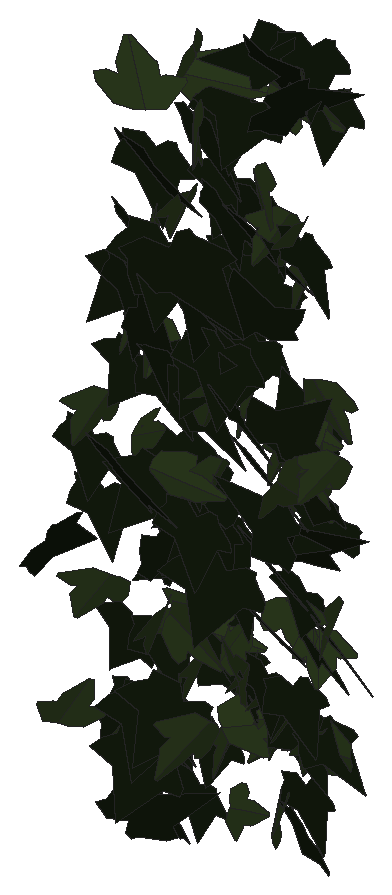
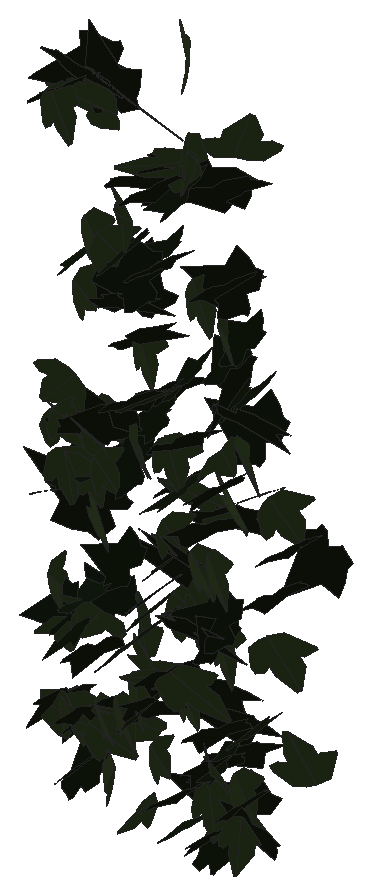
# SketchUp Ruby script. Lengths in inches.
U = 1.inch
M = Sketchup.active_model
def pt(a) = Geom::Point3d.new(a.map { |v| v * U })
def face(e, loops, mat)
  f = e.add_face(loops[0].map { |a| pt(a) })
  loops[1..].each { |l| e.add_face(l.map { |a| pt(a) }).erase! }
  f.material = f.back_material = mat if mat
  f
end
# faces: each face lists its corners as indices into pts; further lists are holes
def faces(e, pts, list, mat = nil) = list.each { |f| face(e, (f[0].is_a?(Array) ? f : [f]).map { |l| l.map { |i| pts[i] } }, mat) }
# xy, xz, yz: faces in a plane at the given z, y or x. An outline is a flat list of corners, or four numbers for a rectangle; further outlines are holes
def ring(l) = l.size == 4 ? [[l[0], l[1]], [l[2], l[1]], [l[2], l[3]], [l[0], l[3]]] : l.each_slice(2).to_a
def flat(e, list, mat, &to3) = list.each { |f| face(e, (f[0].is_a?(Array) ? f : [f]).map { |l| ring(l).map { |u, v| to3.(u, v) } }, mat) }
def xy(e, z, list, mat = nil) = flat(e, list, mat) { |x, y| [x, y, z] }
def xz(e, y, list, mat = nil) = flat(e, list, mat) { |x, z| [x, y, z] }
def yz(e, x, list, mat = nil) = flat(e, list, mat) { |y, z| [x, y, z] }
def lines(e, pts, list) = list.each { |a, b| e.add_line(pt(pts[a]), pt(pts[b])) }
# prism: a flat outline (further loops are holes) pulled along v
def prism(e, loops, v, mat = nil)
  f = face(e, loops, mat); d = Geom::Vector3d.new(v.map { |x| x * U })
  f.pushpull(f.normal.samedirection?(d) ? d.length : -d.length)
end
def box(e, o, s, mat = nil) = prism(e, [[o, [o[0] + s[0], o[1], o[2]], [o[0] + s[0], o[1] + s[1], o[2]], [o[0], o[1] + s[1], o[2]]]], [0, 0, s[2]], mat)
def at(x, y, z, deg = 0) = Geom::Transformation.translation(pt([x, y, z])) * Geom::Transformation.rotation(ORIGIN, Z_AXIS, deg.degrees)
def axes(o, x, y, z) = Geom::Transformation.new([*x, 0, *y, 0, *z, 0, *pt(o).to_a, 1])
def part(name) = M.definitions.add(name)
# library, detail: a bought-in or finely detailed component or shape, given as its bounding box
def library(name, o, s) = part(name).tap { |d| box(d.entities, o, s) }
def detail(e, o, s) = box(e.add_group.entities, o, s)
def put(e, d, t, mat = nil) = e.add_instance(d, t).tap { |i| i.material = mat if mat }
def group(e, t, mat = nil) = e.add_group.tap { |g| g.transformation = t; g.material = mat if mat }.entities
root = M.entities
M.materials.add("1026 AP 7946 SUNNY SIDE UP").color = [254, 231, 186]
M.materials.add("efeu1").color = [18, 25, 13]
M.materials.add("efeu2").color = [43, 57, 29]
c1 = part("ivyleaf_10")
p = [[0,0.5,-0.03],[-0.0625,2.02,-0.43],[-0.19,2.01,-0.46],[-0.54,1.05,-0.29],[-0.52,0.625,-0.18],[-0.83,0.76,-0.28],
  [-1.16,0.64,-0.33],[-1.15,0.33,-0.24],[-0.77,-0.39,0.02],[-0.3,-0.51,0.16],[0.04,-0.48,0.23],[-0.02,2.01,-0.4375],
  [-0.06,2.01,-0.43],[0.04,-0.49,0.23],[0.67,-0.49,0.14],[1.38,0.36,-0.2],[1.375,0.51,-0.24],[0.81,0.65,-0.19],
  [0.62,0.59,-0.15],[0.6,1.09,-0.28],[0.5,1.23,-0.31]]
faces(c1.entities,p,[[0,1,2,3,4,5,6,7,8,9,10],[11,12,0,13,14,15,16,17,18,19,20]],"efeu2")
c2 = part("ivyleaf_9")
p = [[1.54,2.16,1.25],[1.36,2.04,1.19],[-0.21,0.99,0.68],[-0.71,1.11,0.82],[-0.85,0.86,0.67],[-0.8,0.17,0.21],
  [-0.9,-0.01,0.1],[-0.67,-0.16,-0.02],[-0.08,-0.08,-0.05],[-0.03,-0.6,-0.4],[0.65,-0.88,-0.66],[0.83,-0.6,-0.49],
  [1.29,-0.42,-0.43],[1.8125,-0.07,-0.26],[1.21,0.44,0.15]]
faces(c2.entities,p,[[0,1,2,3,4,5,6,7,8,9,10,11,12,13,14]],"efeu1")
put(root,c1,axes([104.9,211.85,273.21],[-0.13637,-0.25929,0.15931],[-0.00882,-0.16099,-0.27962],[0.47582,-0.0773,0.04048]),"1026 AP 7946 SUNNY SIDE UP")
put(root,c2,axes([104.76,211.88,272.62],[-0.08872,-0.27066,0.06287],[-0.00066,-0.06376,-0.28492],[0.43681,-0.05507,0.01234]),"1026 AP 7946 SUNNY SIDE UP")
put(root,c1,axes([104.85,211.24,268.93],[-0.23309,-0.23778,0.08634],[0.05181,0.07969,0.28879],[-0.39375,0.15124,-0.01311]),"1026 AP 7946 SUNNY SIDE UP")
put(root,c2,axes([105.06,212.45,274.85],[-0.44652,-0.06542,-0.02912],[0.05355,-0.02432,-0.29862],[0.09817,-0.2843,0.03048]),"1026 AP 7946 SUNNY SIDE UP")
put(root,c1,axes([105.03,212.42,274.24],[0.21825,-0.25056,0.01931],[-0.00739,-0.02562,-0.29475],[0.39519,0.1379,-0.01618]),"1026 AP 7946 SUNNY SIDE UP")
put(root,c2,axes([104.9375,211.88,271.9],[-0.04719,-0.27806,-0.01852],[0.00454,0.01618,-0.28802],[0.43795,-0.03013,0.00099]),"1026 AP 7946 SUNNY SIDE UP")
put(root,c2,axes([105.04,212.46,273.54],[-0.21801,-0.20803,0.13532],[-0.01162,-0.14847,-0.2489],[0.38767,-0.12144,0.06864]),"1026 AP 7946 SUNNY SIDE UP")
put(root,c1,axes([105.2,211.54,270.84],[-0.2765,-0.20385,0.12948],[-0.11042,-0.10669,-0.27754],[0.36102,-0.18876,0.01429]),"1026 AP 7946 SUNNY SIDE UP")
put(root,c1,axes([105.15,212.29,268.43],[-0.15989,-0.26875,-0.07973],[0.05518,0.0678,-0.2955],[0.43562,-0.10723,0.00817]),"1026 AP 7946 SUNNY SIDE UP")
put(root,c2,axes([105.17,210.46,271.89],[-0.08244,0.06946,-0.3413],[-0.20675,0.30517,0.08904],[0.49112,0.14013,-0.01981]),"1026 AP 7946 SUNNY SIDE UP")
put(root,c2,axes([105.11,212.25,269.82],[-0.12855,-0.20054,0.19397],[-0.03349,-0.19239,-0.22043],[0.43247,-0.07451,0.04059]),"1026 AP 7946 SUNNY SIDE UP")
put(root,c2,axes([105.09,212.36,268.85],[0.03221,-0.26751,-0.0102],[-0.01043,0.0079,-0.27627],[0.4207,0.02068,-0.00607]),"1026 AP 7946 SUNNY SIDE UP")
put(root,c2,axes([105.14,212.16,274.92],[0.02183,-0.27141,0.12572],[0.00089,-0.12368,-0.28064],[0.46892,0.01287,-0.00532]),"1026 AP 7946 SUNNY SIDE UP")
put(root,c2,axes([105.0625,212.2,268.5],[-0.13577,-0.09502,-0.25981],[0.39493,0.06615,-0.11412],[0.15144,-0.2577,0.06469]),"1026 AP 7946 SUNNY SIDE UP")
put(root,c1,axes([105.38,212.03,268.92],[0.00367,-0.26318,0.05046],[0.00058,-0.05047,-0.27143],[0.42137,0.00236,-0.00007]),"1026 AP 7946 SUNNY SIDE UP")
put(root,c1,axes([105.36,212.4375,274.15],[0.09008,0.24911,-0.15821],[-0.05799,-0.15054,-0.26421],[-0.45767,0.06811,0.00234]),"1026 AP 7946 SUNNY SIDE UP")
put(root,c2,axes([105.33,212.42,276.71],[-0.07345,-0.30952,-0.02113],[0.01188,0.01782,-0.32233],[0.48744,-0.04708,0.00468]),"1026 AP 7946 SUNNY SIDE UP")
put(root,c2,axes([105.21,212.15,275.69],[0.09186,-0.2163,0.20667],[0.10874,-0.19006,-0.23155],[0.45231,0.08962,0.0137]),"1026 AP 7946 SUNNY SIDE UP")
put(root,c2,axes([105.14,212.27,276.61],[0.27502,-0.1664,0.2202],[0.20993,-0.16971,-0.24855],[0.37195,0.21882,-0.02254]),"1026 AP 7946 SUNNY SIDE UP")
put(root,c1,axes([105.64,212.27,272.25],[0.0843,-0.28218,-0.00006],[-0.00823,-0.00256,-0.29586],[0.44363,0.05358,-0.00548]),"1026 AP 7946 SUNNY SIDE UP")
put(root,c2,axes([105.4375,212.4375,273.6],[0.05174,-0.275,-0.07016],[0.01303,0.0679,-0.28446],[0.4447,0.03001,0.0165]),"1026 AP 7946 SUNNY SIDE UP")
put(root,c2,axes([105.49,212.38,269.87],[-0.04198,-0.26855,-0.07003],[0.0351,0.06445,-0.27719],[0.43359,-0.03122,0.01566]),"1026 AP 7946 SUNNY SIDE UP")
put(root,c1,axes([105.47,212.28,275.92],[0.17667,-0.18158,0.26379],[0.25223,-0.20184,-0.22026],[0.42582,0.1949,0.02102]),"1026 AP 7946 SUNNY SIDE UP")
put(root,c2,axes([105.48,212.4,268.3125],[0.08229,-0.24938,-0.08234],[0.01437,0.08177,-0.26081],[0.41086,0.04709,0.02562]),"1026 AP 7946 SUNNY SIDE UP")
put(root,c1,axes([105.7,212.25,268.74],[-0.12518,-0.28862,-0.03169],[0.02286,0.0262,-0.3082],[0.45556,-0.08062,0.00676]),"1026 AP 7946 SUNNY SIDE UP")
put(root,c2,axes([105.44,212.18,275.33],[0.03713,-0.23221,0.2238],[0.08523,-0.21305,-0.24047],[0.49412,0.0542,0.02466]),"1026 AP 7946 SUNNY SIDE UP")
put(root,c2,axes([105.6875,212.09,270.97],[-0.11798,-0.09311,0.30162],[0.27453,0.23574,0.12448],[-0.39848,0.18998,-0.00354]),"1026 AP 7946 SUNNY SIDE UP")
put(root,c2,axes([105.35,212.36,271.51],[0.31568,-0.1769,0.16046],[0.15625,-0.12345,-0.27534],[0.33722,0.2228,-0.02264]),"1026 AP 7946 SUNNY SIDE UP")
put(root,c1,axes([105.49,211.9375,272.88],[0.09376,-0.2018,-0.22314],[0.21226,-0.17684,0.20809],[-0.41281,-0.13677,0.05632]),"1026 AP 7946 SUNNY SIDE UP")
put(root,c2,axes([105.74,211.59,274.93],[0.13813,-0.14527,-0.30319],[-0.28903,0.2296,-0.17241],[0.42613,0.20281,-0.01867]),"1026 AP 7946 SUNNY SIDE UP")
put(root,c1,axes([105.79,212.43,272.34],[0.08405,-0.26833,0.06119],[0.00277,-0.06172,-0.28203],[0.43265,0.05252,-0.01008]),"1026 AP 7946 SUNNY SIDE UP")
put(root,c1,axes([105.6,212.35,269.28],[0.27085,-0.11401,0.1883],[0.21361,-0.1252,-0.21233],[0.26401,0.21827,-0.02138]),"1026 AP 7946 SUNNY SIDE UP")
put(root,c2,axes([105.88,212.01,267.58],[0.20182,-0.28633,0.03714],[-0.00612,0.03951,0.32323],[-0.45406,-0.1278,0.01215]),"1026 AP 7946 SUNNY SIDE UP")
put(root,c1,axes([105.875,211.44,278.15],[0.38142,0.24059,0.01396],[-0.04199,0.00967,0.35102],[0.37645,-0.24268,0.02501]),"1026 AP 7946 SUNNY SIDE UP")
put(root,c1,axes([106.1875,212.32,270.33],[-0.25609,-0.06799,0.2564],[-0.33715,-0.12884,-0.18128],[0.22668,-0.26844,0.02004]),"1026 AP 7946 SUNNY SIDE UP")
put(root,c2,axes([106.11,212.41,271.28],[-0.45539,-0.01295,0.03436],[-0.05016,-0.03104,-0.2973],[0.02572,-0.28988,0.02858]),"1026 AP 7946 SUNNY SIDE UP")
put(root,c1,axes([105.9375,212.24,276.3125],[-0.00814,-0.29914,0.02278],[0.00021,-0.02382,-0.30835],[0.47185,-0.00515,0.00053]),"1026 AP 7946 SUNNY SIDE UP")
put(root,c2,axes([105.6875,211.99,269.13],[0.23262,-0.22919,-0.01236],[-0.02358,0.00304,-0.28078],[0.36,0.14829,-0.01041]),"1026 AP 7946 SUNNY SIDE UP")
put(root,c2,axes([105.71,211.8125,274.46],[0.10779,-0.26528,0.10233],[0.0118,-0.10201,-0.28231],[0.44609,0.0668,-0.01726]),"1026 AP 7946 SUNNY SIDE UP")
put(root,c2,axes([105.8,212.02,269.1],[0.00751,-0.25154,-0.10071],[0.02049,0.09645,-0.25822],[0.42304,-0.0002,0.01429]),"1026 AP 7946 SUNNY SIDE UP")
put(root,c2,axes([105.82,212.24,272.8],[-0.05672,-0.26808,-0.09466],[0.06542,0.08507,-0.27663],[0.44,-0.04721,0.02893]),"1026 AP 7946 SUNNY SIDE UP")
put(root,c2,axes([106.125,211.58,272.6],[-0.37623,-0.18071,0.05784],[-0.04976,-0.05269,-0.30833],[0.29385,-0.2403,0.02184]),"1026 AP 7946 SUNNY SIDE UP")
put(root,c1,axes([106.11,211.54,270.7],[0.04765,-0.33136,-0.03264],[-0.01071,0.0293,-0.34259],[0.52302,0.03079,-0.00404]),"1026 AP 7946 SUNNY SIDE UP")
put(root,c1,axes([106.07,212.23,278.49],[0.0481,-0.28273,-0.13279],[0.06871,0.13057,-0.28717],[0.48268,0.00959,0.05411]),"1026 AP 7946 SUNNY SIDE UP")
put(root,c2,axes([106.15,211.26,268.79],[-0.26122,-0.27364,0.06493],[-0.0318,-0.06319,-0.32979],[0.44095,-0.16667,0.01468]),"1026 AP 7946 SUNNY SIDE UP")
put(root,c2,axes([106.2,211.4,269.43],[-0.41224,-0.17388,-0.09526],[0.14983,0.02088,-0.32208],[0.27017,-0.27689,0.03327]),"1026 AP 7946 SUNNY SIDE UP")
put(root,c2,axes([106.22,212.39,274],[-0.21257,-0.24818,0.0884],[-0.0298,-0.08862,-0.29056],[0.41256,-0.13427,0.02456]),"1026 AP 7946 SUNNY SIDE UP")
put(root,c2,axes([106.02,212.4,273.36],[0.21197,-0.25152,-0.06967],[-0.00573,0.07273,-0.2919],[0.40892,0.1314,0.03202]),"1026 AP 7946 SUNNY SIDE UP")
put(root,c2,axes([106.53,212.28,272.32],[-0.49536,0.04052,-0.00725],[0.00486,-0.03261,-0.32575],[-0.06454,-0.31343,0.03107]),"1026 AP 7946 SUNNY SIDE UP")
put(root,c2,axes([105.99,211.12,267.89],[0.01157,0.00502,0.33337],[0.50166,0.05409,-0.00802],[-0.08522,0.3191,-0.00196]),"1026 AP 7946 SUNNY SIDE UP")
put(root,c2,axes([106.24,212.53,268.6],[-0.11135,-0.23911,0.07407],[-0.0032,-0.07559,-0.25662],[0.39321,-0.06833,0.01889]),"1026 AP 7946 SUNNY SIDE UP")
put(root,c2,axes([106.21,212.21,274.82],[-0.016,-0.23467,0.22372],[-0.01108,-0.21839,-0.24325],[0.50405,-0.01225,0.00175]),"1026 AP 7946 SUNNY SIDE UP")
put(root,c2,axes([106.25,212.15,267.99],[-0.05486,-0.24507,0.10833],[0.02508,-0.10917,-0.25394],[0.41943,-0.02552,0.02935]),"1026 AP 7946 SUNNY SIDE UP")
put(root,c1,axes([106.4,211.97,269.9375],[0.06799,-0.2653,0.06896],[0.02081,-0.06719,-0.2773],[0.43031,0.04517,0.00251]),"1026 AP 7946 SUNNY SIDE UP")
put(root,c1,axes([106.45,212.2,273.74],[-0.11432,-0.2791,0.02523],[0.00059,-0.02704,-0.29719],[0.44077,-0.07236,0.00694]),"1026 AP 7946 SUNNY SIDE UP")
put(root,c1,axes([106.4,212.28,272.5625],[-0.04556,-0.24319,0.14883],[0.06393,-0.14866,-0.2479],[0.44128,-0.00357,0.05128]),"1026 AP 7946 SUNNY SIDE UP")
put(root,c2,axes([106.38,212.35,270.42],[-0.0352,-0.26991,-0.06468],[0.0018,0.06136,-0.27862],[0.43519,-0.02208,-0.00408]),"1026 AP 7946 SUNNY SIDE UP")
put(root,c2,axes([106.29,212.04,277.66],[0.25695,-0.28729,0.00723],[-0.01279,-0.01457,-0.34026],[0.45176,0.16299,-0.01375]),"1026 AP 7946 SUNNY SIDE UP")
put(root,c1,axes([106.22,212.22,278.17],[-0.0047,-0.11737,-0.3196],[0.45124,0.15345,-0.0619],[0.25959,-0.26888,0.10181]),"1026 AP 7946 SUNNY SIDE UP")
put(root,c2,axes([106.49,212.55,276.63],[-0.15166,-0.26073,0.10988],[-0.02607,-0.10885,-0.28624],[0.44308,-0.09565,0.02077]),"1026 AP 7946 SUNNY SIDE UP")
put(root,c1,axes([106.18,211.59,272.72],[-0.03081,-0.07645,-0.30464],[0.45752,-0.09345,0.00449],[-0.14388,-0.28079,0.0795]),"1026 AP 7946 SUNNY SIDE UP")
put(root,c2,axes([106.64,211.29,269.71],[-0.46195,-0.14833,-0.03599],[0.06836,-0.01077,-0.33778],[0.22934,-0.29556,0.0282]),"1026 AP 7946 SUNNY SIDE UP")
put(root,c2,axes([106.17,210.57,273.24],[0.19293,-0.21382,0.28291],[0.24666,-0.2274,-0.25481],[0.49021,0.19857,0.01687]),"1026 AP 7946 SUNNY SIDE UP")
put(root,c1,axes([106.29,212.16,270.29],[-0.07172,-0.10114,-0.27861],[0.42734,0.07584,-0.07616],[0.15081,-0.26298,0.08329]),"1026 AP 7946 SUNNY SIDE UP")
put(root,c2,axes([106.46,212.49,271.67],[0.04829,-0.28427,0.01373],[-0.0028,-0.01522,-0.29462],[0.44759,0.03057,-0.00333]),"1026 AP 7946 SUNNY SIDE UP")
put(root,c2,axes([106.47,212.5,271.15],[0.04577,-0.27563,0.05457],[-0.00146,-0.05492,-0.28577],[0.4418,0.02837,-0.0066]),"1026 AP 7946 SUNNY SIDE UP")
put(root,c2,axes([106.55,212.48,277.78],[-0.10833,-0.29768,0.04135],[-0.00512,-0.04217,-0.31495],[0.47264,-0.06868,0.00607]),"1026 AP 7946 SUNNY SIDE UP")
put(root,c2,axes([106.78,212.59,275.48],[-0.27231,-0.16149,0.17914],[-0.15479,-0.14822,-0.2424],[0.3407,-0.19642,0.03305]),"1026 AP 7946 SUNNY SIDE UP")
put(root,c2,axes([106.62,212.58,274.54],[-0.1738,-0.22256,0.15327],[0.01058,-0.16451,-0.24725],[0.42192,-0.08755,0.06933]),"1026 AP 7946 SUNNY SIDE UP")
put(root,c2,axes([106.52,212.09,271.97],[0.07228,-0.27799,0.01967],[-0.00116,-0.02107,-0.29037],[0.43832,0.04579,-0.00401]),"1026 AP 7946 SUNNY SIDE UP")
put(root,c2,axes([106.52,212.35,269.9],[0.00219,-0.22481,-0.16551],[0.10086,0.15527,-0.22413],[0.42141,-0.036,0.05451]),"1026 AP 7946 SUNNY SIDE UP")
put(root,c1,axes([106.4,211.53,270.64],[0.12286,0.00441,0.3361],[0.50022,-0.07545,-0.07788],[0.11381,0.32686,-0.0205]),"1026 AP 7946 SUNNY SIDE UP")
put(root,c1,axes([106.74,212.11,268.94],[0.0522,-0.22051,0.15706],[0.09888,-0.14421,-0.22796],[0.41093,0.06271,0.03491]),"1026 AP 7946 SUNNY SIDE UP")
put(root,c1,axes([106.85,212.26,275.22],[0.01345,-0.2958,-0.01911],[0.00236,0.01692,-0.30476],[0.46587,0.00845,0.0021]),"1026 AP 7946 SUNNY SIDE UP")
put(root,c2,axes([106.73,212.04,274.47],[-0.15201,-0.32331,0.01322],[0.00756,-0.01674,-0.3476],[0.50883,-0.09633,0.00912]),"1026 AP 7946 SUNNY SIDE UP")
put(root,c2,axes([106.82,212.44,277.875],[-0.24512,-0.26249,0.04735],[-0.00976,-0.05138,-0.31409],[0.41932,-0.15464,0.02037]),"1026 AP 7946 SUNNY SIDE UP")
put(root,c2,axes([106.69,212.52,269.76],[0.05466,-0.24955,0.08426],[0.00451,-0.08357,-0.25992],[0.41361,0.03389,-0.0083]),"1026 AP 7946 SUNNY SIDE UP")
put(root,c1,axes([106.81,212.46,273.77],[0.25219,-0.21977,0.11671],[0.09951,-0.09559,-0.2808],[0.37676,0.17235,-0.00396]),"1026 AP 7946 SUNNY SIDE UP")
put(root,c2,axes([106.7,212.1,276.5],[0.05573,-0.26159,0.15517],[0.04479,-0.14959,-0.27272],[0.47369,0.04492,0.00753]),"1026 AP 7946 SUNNY SIDE UP")
put(root,c2,axes([106.74,212.29,271.16],[0.04401,-0.27695,0.06206],[-0.0028,-0.06228,-0.28702],[0.44619,0.02693,-0.00792]),"1026 AP 7946 SUNNY SIDE UP")
put(root,c1,axes([106.76,212.1,270.1],[0.36354,-0.1687,-0.06823],[0.10768,-0.01641,0.29349],[-0.26326,-0.23968,0.02583]),"1026 AP 7946 SUNNY SIDE UP")
put(root,c2,axes([106.9,212.49,274.44],[-0.19493,-0.26391,0.05475],[-0.00279,-0.05934,-0.29977],[0.42377,-0.12179,0.02321]),"1026 AP 7946 SUNNY SIDE UP")
put(root,c1,axes([107,212.2,269.95],[0.02677,-0.27688,-0.06305],[-0.00701,0.05947,-0.28543],[0.4453,0.01758,-0.0007]),"1026 AP 7946 SUNNY SIDE UP")
put(root,c1,axes([106.98,211.97,268.02],[0.06046,-0.14081,-0.23688],[0.15914,0.22203,-0.12177],[0.3918,-0.06845,0.08601]),"1026 AP 7946 SUNNY SIDE UP")
put(root,c2,axes([106.85,211.85,273.97],[0.30936,-0.21329,-0.00151],[-0.00817,-0.00444,-0.29887],[0.33528,0.19669,-0.00588]),"1026 AP 7946 SUNNY SIDE UP")
put(root,c1,axes([107.14,212.36,269.6],[0.07173,-0.26739,0.00927],[-0.00657,-0.01138,-0.27944],[0.42072,0.04541,-0.00594]),"1026 AP 7946 SUNNY SIDE UP")
put(root,c2,axes([107.04,210.52,276.76],[-0.22038,-0.33105,-0.00628],[0.02151,-0.00122,-0.37011],[0.52014,-0.14021,0.01264]),"1026 AP 7946 SUNNY SIDE UP")
put(root,c2,axes([107.14,211.53,271.65],[-0.43131,-0.17347,-0.09423],[0.14399,0.02388,-0.33299],[0.27187,-0.28785,0.02686]),"1026 AP 7946 SUNNY SIDE UP")
put(root,c2,axes([107.47,212.17,278.9],[-0.3723,0.18073,0.08973],[-0.15982,0.0063,-0.30166],[-0.27117,-0.25185,0.0546]),"1026 AP 7946 SUNNY SIDE UP")
put(root,c2,axes([107.04,211.1,272.58],[-0.07848,-0.30433,0.03796],[-0.00204,-0.03887,-0.31789],[0.48235,-0.04968,0.00483]),"1026 AP 7946 SUNNY SIDE UP")
put(root,c2,axes([106.81,212.25,276.21],[0.36962,-0.17414,0.14887],[0.16247,-0.10437,-0.30128],[0.31767,0.25599,-0.01913]),"1026 AP 7946 SUNNY SIDE UP")
put(root,c2,axes([107.08,212.36,276.58],[0.10079,-0.29443,0.04408],[0.00425,-0.0449,-0.31061],[0.4682,0.06379,-0.00667]),"1026 AP 7946 SUNNY SIDE UP")
put(root,c1,axes([106.99,212,269.21],[0.19479,-0.03689,-0.27072],[0.40072,0.0966,0.11045],[0.11514,-0.27379,0.07361]),"1026 AP 7946 SUNNY SIDE UP")
put(root,c2,axes([107.5,212.19,275.64],[-0.38722,-0.12558,0.11413],[-0.11613,-0.09676,-0.28087],[0.23715,-0.25242,0.04882]),"1026 AP 7946 SUNNY SIDE UP")
put(root,c1,axes([107.18,212.23,276.99],[-0.15396,0.1095,-0.28686],[0.16897,-0.26126,-0.14597],[-0.44007,-0.13863,0.04431]),"1026 AP 7946 SUNNY SIDE UP")
put(root,c1,axes([107.49,212.37,269.14],[-0.08411,-0.18967,0.20499],[-0.08254,-0.19306,-0.20415],[0.42555,-0.07493,0.00092]),"1026 AP 7946 SUNNY SIDE UP")
put(root,c1,axes([107.42,212.45,273.25],[0.00648,-0.24113,0.15371],[0.06566,-0.14844,-0.24694],[0.44216,0.02558,0.03442]),"1026 AP 7946 SUNNY SIDE UP")
put(root,c1,axes([107.5,212.23,276.52],[-0.12256,-0.21633,0.20035],[0.0148,-0.20433,-0.23001],[0.45846,-0.05123,0.06099]),"1026 AP 7946 SUNNY SIDE UP")
put(root,c1,axes([107.32,211.58,270.17],[-0.29148,0.16356,0.21147],[0.27746,-0.10685,0.25239],[0.30397,0.25437,-0.02759]),"1026 AP 7946 SUNNY SIDE UP")
put(root,c2,axes([107.16,212,273.14],[0.33807,-0.23303,0.0883],[0.07394,-0.07489,-0.32668],[0.38409,0.21953,-0.01483]),"1026 AP 7946 SUNNY SIDE UP")
put(root,c2,axes([107.18,212.1875,271.67],[0.20779,-0.19705,0.18628],[0.14905,-0.15542,-0.24524],[0.3945,0.16251,-0.00546]),"1026 AP 7946 SUNNY SIDE UP")
put(root,c1,axes([107.34,212.54,272.28],[0.07023,-0.17925,-0.24459],[0.15759,-0.2159,0.18689],[-0.43907,-0.10616,0.02796]),"1026 AP 7946 SUNNY SIDE UP")
put(root,c1,axes([107.5625,212.24,269.36],[0.13987,-0.2662,0.03321],[0.00394,-0.03473,-0.28921],[0.42191,0.08857,-0.00831]),"1026 AP 7946 SUNNY SIDE UP")
put(root,c2,axes([107.61,211.58,275.31],[0.33053,0.08483,0.22779],[-0.36192,0.00621,0.22349],[0.08465,-0.30468,0.06605]),"1026 AP 7946 SUNNY SIDE UP")
put(root,c2,axes([107.29,210.3,276.87],[-0.11053,-0.18579,-0.34052],[0.28334,0.27821,-0.19959],[0.52295,-0.19,0.03617]),"1026 AP 7946 SUNNY SIDE UP")
put(root,c1,axes([107.45,210.61,278.63],[-0.06716,0.08857,-0.36025],[0.10715,-0.34433,-0.10029],[-0.55779,-0.07681,0.02411]),"1026 AP 7946 SUNNY SIDE UP")
put(root,c1,axes([107.7,210.3,270.11],[-0.11889,-0.26649,0.24995],[-0.03691,-0.24528,-0.28474],[0.5671,-0.07183,0.03387]),"1026 AP 7946 SUNNY SIDE UP")
put(root,c2,axes([107.52,211.93,270.12],[0.0041,-0.25925,0.09778],[-0.00568,-0.09641,-0.26761],[0.43486,0.00118,-0.00442]),"1026 AP 7946 SUNNY SIDE UP")
put(root,c1,axes([107.82,211.76,268.14],[0.11754,-0.06151,0.32416],[-0.2891,0.25691,0.09813],[-0.41366,-0.19703,0.02353]),"1026 AP 7946 SUNNY SIDE UP")
put(root,c1,axes([107.54,212.35,270.89],[0.39006,0.05363,0.13389],[0.20664,0.00351,-0.26048],[-0.07734,0.27989,-0.02069]),"1026 AP 7946 SUNNY SIDE UP")
put(root,c2,axes([107.57,212.08,278.64],[-0.18477,-0.04313,0.32092],[0.23891,-0.2992,0.01461],[0.43339,0.14655,0.12876]),"1026 AP 7946 SUNNY SIDE UP")
put(root,c2,axes([107.95,212.24,273.48],[-0.43204,-0.10691,0.0776],[0.11042,0.02893,0.3039],[-0.17414,0.28359,0.00017]),"1026 AP 7946 SUNNY SIDE UP")
put(root,c2,axes([107.67,212.51,271.12],[-0.0823,-0.21917,0.16899],[0.05144,-0.17204,-0.22536],[0.42856,-0.02144,0.05951]),"1026 AP 7946 SUNNY SIDE UP")
put(root,c1,axes([107.75,212.47,275.86],[0.05448,-0.22581,0.20382],[0.12332,-0.18675,-0.23332],[0.45705,0.07731,0.03866]),"1026 AP 7946 SUNNY SIDE UP")
put(root,c1,axes([107.85,212.11,276.58],[0.054,-0.29916,0.0581],[0.00698,-0.05796,-0.31055],[0.47914,0.03456,-0.00202]),"1026 AP 7946 SUNNY SIDE UP")
put(root,c2,axes([107.71,212.32,269.39],[0.01889,-0.2731,-0.11938],[-0.01381,0.11405,-0.28093],[0.46533,0.01447,-0.00349]),"1026 AP 7946 SUNNY SIDE UP")
put(root,c2,axes([107.6,211.95,270.76],[0.00565,-0.15347,0.24296],[0.20283,-0.20964,-0.14327],[0.3945,0.10998,0.07018]),"1026 AP 7946 SUNNY SIDE UP")
put(root,c2,axes([107.68,211.95,273.56],[-0.22169,0.06358,0.25449],[0.3663,-0.08187,0.15843],[0.16204,0.27207,-0.00998]),"1026 AP 7946 SUNNY SIDE UP")
put(root,c1,axes([107.74,212.33,272.98],[-0.3482,0.0772,-0.18337],[0.22475,-0.11869,-0.23633],[-0.20723,-0.25844,0.0518]),"1026 AP 7946 SUNNY SIDE UP")
put(root,c1,axes([107.65,212.36,273.52],[0.0075,-0.14293,-0.27585],[0.38095,-0.15835,0.09088],[-0.28562,-0.21496,0.11397]),"1026 AP 7946 SUNNY SIDE UP")
put(root,c2,axes([107.84,212.31,270.71],[0.31575,-0.17394,-0.111],[-0.13187,0.06621,-0.27326],[0.29257,0.21757,-0.00338]),"1026 AP 7946 SUNNY SIDE UP")
put(root,c2,axes([107.8125,212.26,276.3125],[0.12105,-0.29109,0.01569],[-0.00449,-0.01821,-0.3102],[0.45846,0.07668,-0.00718]),"1026 AP 7946 SUNNY SIDE UP")
put(root,c2,axes([107.86,212.28,268.48],[0.05498,-0.2681,0.00417],[-0.00558,-0.00608,-0.27854],[0.42162,0.03488,-0.00423]),"1026 AP 7946 SUNNY SIDE UP")
put(root,c2,axes([108.22,211.38,272.64],[-0.08166,-0.34517,0.0099],[0.007,0.01103,0.35965],[-0.54301,0.05205,0.00315]),"1026 AP 7946 SUNNY SIDE UP")
put(root,c1,axes([108.37,212.29,269.15],[-0.03164,0.03068,0.29327],[-0.4472,-0.03358,-0.01719],[0.04959,-0.28322,0.0321]),"1026 AP 7946 SUNNY SIDE UP")
put(root,c1,axes([108.09,212.23,269.3],[-0.01844,-0.28134,0.03439],[-0.00124,-0.03498,-0.29029],[0.44579,-0.01173,0.00062]),"1026 AP 7946 SUNNY SIDE UP")
put(root,c2,axes([107.91,212.32,279.11],[-0.31078,-0.14681,-0.19216],[0.33419,-0.00352,-0.23019],[0.16391,-0.27117,0.10497]),"1026 AP 7946 SUNNY SIDE UP")
put(root,c1,axes([108.11,212.32,273.05],[-0.19397,-0.26272,0.00652],[0.00655,-0.01059,-0.29894],[0.41323,-0.12315,0.0078]),"1026 AP 7946 SUNNY SIDE UP")
put(root,c1,axes([107.64,212.1,278.48],[0.03462,0.02157,0.35833],[0.54768,0.00519,-0.02302],[-0.0103,0.34836,-0.01979]),"1026 AP 7946 SUNNY SIDE UP")
put(root,c2,axes([107.9375,211.93,270.08],[0.00193,-0.26077,-0.09815],[-0.01181,0.09372,-0.26801],[0.43558,0.0037,-0.00683]),"1026 AP 7946 SUNNY SIDE UP")
put(root,c1,axes([108.03,212.34,270.62],[0.22838,0.23179,-0.04251],[-0.01905,-0.04261,-0.28176],[-0.37007,0.14523,-0.01173]),"1026 AP 7946 SUNNY SIDE UP")
put(root,c1,axes([108.07,212.52,273.84],[-0.10031,-0.17281,0.22779],[0.15379,-0.22715,-0.15446],[0.4149,0.04242,0.11233]),"1026 AP 7946 SUNNY SIDE UP")
put(root,c2,axes([108.03,212.27,272.78],[-0.13011,-0.18556,0.20905],[0.11323,-0.22011,-0.17748],[0.41855,0.00186,0.113]),"1026 AP 7946 SUNNY SIDE UP")
put(root,c2,axes([108.02,211.44,278.7],[0.03358,0.19515,-0.30772],[-0.0388,0.30044,0.20141],[0.56116,0.00909,0.03234]),"1026 AP 7946 SUNNY SIDE UP")
put(root,c1,axes([108.15,211.4,273.35],[-0.07749,-0.23044,-0.26837],[0.12167,0.24789,-0.24075],[0.53159,-0.09033,0.01598]),"1026 AP 7946 SUNNY SIDE UP")
put(root,c2,axes([107.82,211.86,272.21],[0.42379,0.12316,-0.1537],[0.19068,0.09332,0.30417],[0.23812,-0.29394,0.02997]),"1026 AP 7946 SUNNY SIDE UP")
put(root,c1,axes([108.27,212.35,278.49],[-0.05224,-0.30044,0.04798],[-0.00246,-0.0484,-0.31166],[0.47847,-0.03305,0.00364]),"1026 AP 7946 SUNNY SIDE UP")
put(root,c2,axes([108.1,212.01,267.97],[-0.10447,-0.11095,0.28564],[0.05814,-0.28553,-0.11],[0.46689,0.01073,0.07761]),"1026 AP 7946 SUNNY SIDE UP")
put(root,c1,axes([108.12,212.31,274.26],[-0.37416,0.0844,-0.15447],[0.18699,-0.10536,-0.25532],[-0.19644,-0.26105,0.05117]),"1026 AP 7946 SUNNY SIDE UP")
put(root,c2,axes([108.34,212.29,272.49],[-0.29596,-0.16536,0.142],[-0.03495,-0.1683,-0.23863],[0.33765,-0.16237,0.09977]),"1026 AP 7946 SUNNY SIDE UP")
put(root,c2,axes([108.18,212.2,269.41],[0.07981,-0.21204,-0.17232],[-0.00954,0.16804,-0.22198],[0.42339,0.04376,0.02748]),"1026 AP 7946 SUNNY SIDE UP")
put(root,c1,axes([108.46,212.04,273.43],[-0.16072,-0.19796,0.19067],[-0.04013,-0.19107,-0.22481],[0.42544,-0.0928,0.05083]),"1026 AP 7946 SUNNY SIDE UP")
put(root,c2,axes([108.11,212.33,270.81],[0.29526,-0.19596,0.05871],[0.03764,-0.05727,-0.27903],[0.31918,0.18803,-0.02141]),"1026 AP 7946 SUNNY SIDE UP")
put(root,c2,axes([108.27,212.23,278.63],[-0.11453,-0.29871,0.0466],[0.01365,-0.05032,-0.31636],[0.47526,-0.07054,0.02032]),"1026 AP 7946 SUNNY SIDE UP")
put(root,c1,axes([108.31,212.31,271.15],[0.10587,-0.18717,0.22501],[0.14706,-0.19903,-0.20558],[0.42905,0.1144,0.01494]),"1026 AP 7946 SUNNY SIDE UP")
